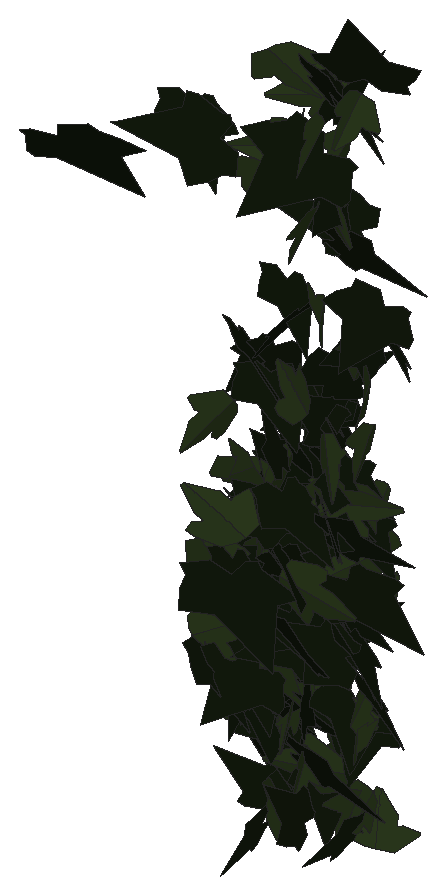
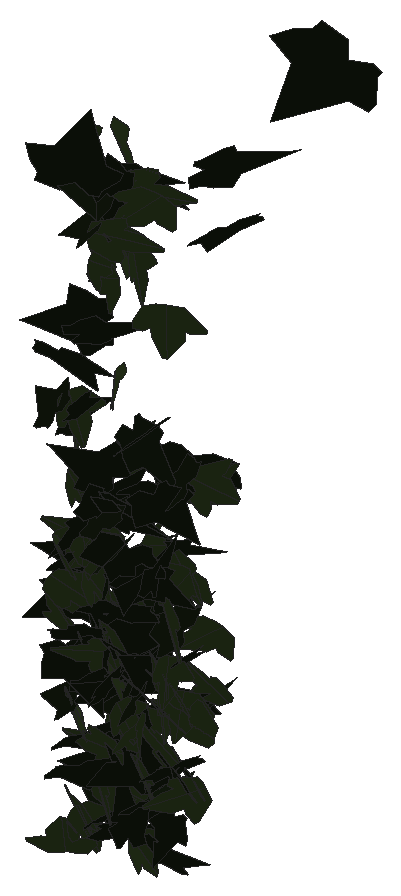
# SketchUp Ruby script. Lengths in inches.
U = 1.inch
M = Sketchup.active_model
def pt(a) = Geom::Point3d.new(a.map { |v| v * U })
def face(e, loops, mat)
  f = e.add_face(loops[0].map { |a| pt(a) })
  loops[1..].each { |l| e.add_face(l.map { |a| pt(a) }).erase! }
  f.material = f.back_material = mat if mat
  f
end
# faces: each face lists its corners as indices into pts; further lists are holes
def faces(e, pts, list, mat = nil) = list.each { |f| face(e, (f[0].is_a?(Array) ? f : [f]).map { |l| l.map { |i| pts[i] } }, mat) }
# xy, xz, yz: faces in a plane at the given z, y or x. An outline is a flat list of corners, or four numbers for a rectangle; further outlines are holes
def ring(l) = l.size == 4 ? [[l[0], l[1]], [l[2], l[1]], [l[2], l[3]], [l[0], l[3]]] : l.each_slice(2).to_a
def flat(e, list, mat, &to3) = list.each { |f| face(e, (f[0].is_a?(Array) ? f : [f]).map { |l| ring(l).map { |u, v| to3.(u, v) } }, mat) }
def xy(e, z, list, mat = nil) = flat(e, list, mat) { |x, y| [x, y, z] }
def xz(e, y, list, mat = nil) = flat(e, list, mat) { |x, z| [x, y, z] }
def yz(e, x, list, mat = nil) = flat(e, list, mat) { |y, z| [x, y, z] }
def lines(e, pts, list) = list.each { |a, b| e.add_line(pt(pts[a]), pt(pts[b])) }
# prism: a flat outline (further loops are holes) pulled along v
def prism(e, loops, v, mat = nil)
  f = face(e, loops, mat); d = Geom::Vector3d.new(v.map { |x| x * U })
  f.pushpull(f.normal.samedirection?(d) ? d.length : -d.length)
end
def box(e, o, s, mat = nil) = prism(e, [[o, [o[0] + s[0], o[1], o[2]], [o[0] + s[0], o[1] + s[1], o[2]], [o[0], o[1] + s[1], o[2]]]], [0, 0, s[2]], mat)
def at(x, y, z, deg = 0) = Geom::Transformation.translation(pt([x, y, z])) * Geom::Transformation.rotation(ORIGIN, Z_AXIS, deg.degrees)
def axes(o, x, y, z) = Geom::Transformation.new([*x, 0, *y, 0, *z, 0, *pt(o).to_a, 1])
def part(name) = M.definitions.add(name)
# library, detail: a bought-in or finely detailed component or shape, given as its bounding box
def library(name, o, s) = part(name).tap { |d| box(d.entities, o, s) }
def detail(e, o, s) = box(e.add_group.entities, o, s)
def put(e, d, t, mat = nil) = e.add_instance(d, t).tap { |i| i.material = mat if mat }
def group(e, t, mat = nil) = e.add_group.tap { |g| g.transformation = t; g.material = mat if mat }.entities
root = M.entities
M.materials.add("1026 AP 7946 SUNNY SIDE UP").color = [254, 231, 186]
M.materials.add("efeu1").color = [18, 25, 13]
M.materials.add("efeu2").color = [43, 57, 29]
c1 = part("ivyleaf_9")
p = [[1.54,2.16,1.25],[1.36,2.04,1.19],[-0.21,0.99,0.68],[-0.71,1.11,0.82],[-0.85,0.86,0.67],[-0.8,0.17,0.21],
  [-0.9,-0.01,0.1],[-0.67,-0.16,-0.02],[-0.08,-0.08,-0.05],[-0.03,-0.6,-0.4],[0.65,-0.88,-0.66],[0.83,-0.6,-0.49],
  [1.29,-0.42,-0.43],[1.8125,-0.07,-0.26],[1.21,0.44,0.15]]
faces(c1.entities,p,[[0,1,2,3,4,5,6,7,8,9,10,11,12,13,14]],"efeu1")
c2 = part("ivyleaf_10")
p = [[0,0.5,-0.03],[-0.0625,2.02,-0.43],[-0.19,2.01,-0.46],[-0.54,1.05,-0.29],[-0.52,0.625,-0.18],[-0.83,0.76,-0.28],
  [-1.16,0.64,-0.33],[-1.15,0.33,-0.24],[-0.77,-0.39,0.02],[-0.3,-0.51,0.16],[0.04,-0.48,0.23],[-0.02,2.01,-0.4375],
  [-0.06,2.01,-0.43],[0.04,-0.49,0.23],[0.67,-0.49,0.14],[1.38,0.36,-0.2],[1.375,0.51,-0.24],[0.81,0.65,-0.19],
  [0.62,0.59,-0.15],[0.6,1.09,-0.28],[0.5,1.23,-0.31]]
faces(c2.entities,p,[[0,1,2,3,4,5,6,7,8,9,10],[11,12,0,13,14,15,16,17,18,19,20]],"efeu2")
put(root,c1,axes([119.4375,207.16,279.6],[0.64011,0.19649,0.04423],[0.08407,-0.01489,-0.46425],[-0.30449,0.40896,-0.03521]),"1026 AP 7946 SUNNY SIDE UP")
put(root,c1,axes([121.18,208.625,272.82],[-0.2498,-0.24915,-0.28445],[0.28289,0.20954,-0.30176],[0.50992,-0.2383,0.02806]),"1026 AP 7946 SUNNY SIDE UP")
put(root,c1,axes([120,209.72,278.67],[-0.11484,-0.29306,-0.27056],[-0.04005,-0.26135,0.30816],[-0.61573,0.07166,0.03042]),"1026 AP 7946 SUNNY SIDE UP")
put(root,c2,axes([120.375,209.6,272.92],[0.1763,0.27302,0.20783],[-0.16656,-0.172,0.30177],[0.50561,-0.15186,0.02694]),"1026 AP 7946 SUNNY SIDE UP")
put(root,c1,axes([120.57,209.97,268.24],[-0.30854,0.13802,-0.17309],[0.19369,-0.11721,-0.24693],[-0.28291,-0.23078,0.01971]),"1026 AP 7946 SUNNY SIDE UP")
put(root,c1,axes([121.38,209.85,268.64],[-0.23324,0.03837,-0.26203],[-0.39193,0.05209,0.15802],[0.10126,0.28999,0.00807]),"1026 AP 7946 SUNNY SIDE UP")
put(root,c2,axes([121.3,210.23,278.98],[0.25906,-0.33094,0.02563],[-0.00335,-0.03092,-0.38068],[0.52205,0.16402,-0.01516]),"1026 AP 7946 SUNNY SIDE UP")
put(root,c1,axes([121.22,210.41,278.53],[-0.6117,-0.16424,0.04847],[-0.04205,-0.05935,-0.433],[0.26574,-0.38745,0.04306]),"1026 AP 7946 SUNNY SIDE UP")
put(root,c1,axes([120.72,210.45,270.88],[0.44713,-0.21603,-0.03017],[0.07123,0.01351,0.36588],[-0.33506,-0.28542,0.03753]),"1026 AP 7946 SUNNY SIDE UP")
put(root,c2,axes([119.36,210.64,273.88],[-0.05934,-0.20383,0.30376],[0.01008,-0.29797,-0.21228],[0.56504,-0.01609,0.03569]),"1026 AP 7946 SUNNY SIDE UP")
put(root,c1,axes([118.96,210.57,278.4],[-0.01902,-0.35708,-0.05764],[0.02386,0.0534,-0.36751],[0.56734,-0.01421,0.01352]),"1026 AP 7946 SUNNY SIDE UP")
put(root,c2,axes([120.8,210.6,278.43],[0.12113,-0.00994,-0.36126],[-0.50129,-0.15168,-0.06861],[-0.22999,0.32536,-0.04071]),"1026 AP 7946 SUNNY SIDE UP")
put(root,c1,axes([119.21,210.53,270.18],[0.23736,-0.30645,-0.08631],[-0.0673,0.07035,-0.35144],[0.49426,0.15674,-0.00641]),"1026 AP 7946 SUNNY SIDE UP")
put(root,c2,axes([120.92,210.58,277.41],[0.12282,-0.35113,0.0529],[0.00072,-0.05452,-0.37071],[0.55845,0.07729,-0.01116]),"1026 AP 7946 SUNNY SIDE UP")
put(root,c1,axes([120.16,210.72,272.51],[-0.31823,-0.07491,0.20229],[-0.24417,-0.13125,-0.21676],[0.22361,-0.24992,0.05121]),"1026 AP 7946 SUNNY SIDE UP")
put(root,c1,axes([119.85,210.78,270.01],[-0.35023,-0.24723,0.12467],[-0.09219,-0.11132,-0.34216],[0.42389,-0.22848,0.02859]),"1026 AP 7946 SUNNY SIDE UP")
put(root,c1,axes([119.58,210.65,271.62],[0.14268,-0.32554,-0.02877],[-0.02831,0.02203,-0.34782],[0.51273,0.09181,-0.0112]),"1026 AP 7946 SUNNY SIDE UP")
put(root,c2,axes([120.18,210.71,268.08],[-0.06528,0.01007,0.34132],[0.46943,-0.14382,0.04221],[0.22626,0.30129,0.01091]),"1026 AP 7946 SUNNY SIDE UP")
put(root,c2,axes([119.07,210.66,270.38],[0.2878,-0.07638,-0.21473],[0.32018,-0.0484,0.20262],[-0.13739,-0.2728,0.0224]),"1026 AP 7946 SUNNY SIDE UP")
put(root,c1,axes([121.5,210.73,268.11],[-0.29188,0.21127,-0.08709],[0.06606,-0.07698,-0.28956],[-0.35238,-0.18943,0.01786]),"1026 AP 7946 SUNNY SIDE UP")
put(root,c1,axes([121.22,210.89,270.65],[-0.19629,-0.25938,-0.14117],[-0.10751,-0.11745,0.2957],[-0.44746,0.142,-0.00912]),"1026 AP 7946 SUNNY SIDE UP")
put(root,c2,axes([121.47,210.93,279.14],[0.1149,0.22617,-0.21797],[-0.11951,-0.19901,-0.24588],[-0.47353,0.10511,0.00916]),"1026 AP 7946 SUNNY SIDE UP")
put(root,c2,axes([120.43,210.94,271.45],[-0.08234,-0.00073,-0.36593],[0.50214,-0.15729,-0.04909],[-0.24453,-0.32275,0.02241]),"1026 AP 7946 SUNNY SIDE UP")
put(root,c2,axes([119.01,210.85,271.5625],[-0.34863,-0.0415,-0.18311],[0.28597,-0.03129,-0.22667],[0.01955,-0.28229,0.05033]),"1026 AP 7946 SUNNY SIDE UP")
put(root,c2,axes([120.5,211.07,268.74],[-0.00229,0.18835,-0.23483],[-0.03553,-0.22843,-0.19472],[-0.4649,0.01653,0.01604]),"1026 AP 7946 SUNNY SIDE UP")
put(root,c1,axes([120.18,211.18,271.46],[0.02218,-0.19522,0.24221],[0.04846,-0.23437,-0.20281],[0.47942,0.03272,0.00929]),"1026 AP 7946 SUNNY SIDE UP")
put(root,c1,axes([120.49,211.01,268.78],[0.41517,-0.14986,0.1736],[0.20888,-0.10793,-0.31236],[0.28779,0.29454,-0.02373]),"1026 AP 7946 SUNNY SIDE UP")
put(root,c1,axes([120.17,211,272.71],[0.10327,-0.28964,-0.14862],[0.0423,0.14994,-0.30007],[0.50588,0.04659,0.05543]),"1026 AP 7946 SUNNY SIDE UP")
put(root,c1,axes([120.79,211.26,277.42],[-0.05716,-0.2167,0.2424],[-0.07041,-0.23229,-0.22769],[0.49947,-0.05755,-0.00435]),"1026 AP 7946 SUNNY SIDE UP")
put(root,c1,axes([120.33,210.96,270.93],[-0.04795,-0.1826,-0.27679],[0.16866,0.24798,-0.18543],[0.48073,-0.10521,0.03745]),"1026 AP 7946 SUNNY SIDE UP")
put(root,c1,axes([120.6,210.89,269.82],[0.13315,-0.0998,-0.30264],[-0.38165,0.16745,-0.12995],[0.30254,0.25515,-0.03073]),"1026 AP 7946 SUNNY SIDE UP")
put(root,c1,axes([120.33,211.26,270.32],[-0.32033,-0.06908,0.19298],[-0.23628,-0.12399,-0.21573],[0.20759,-0.24772,0.05224]),"1026 AP 7946 SUNNY SIDE UP")
put(root,c2,axes([120.28,211.14,274.1],[-0.12262,0.3353,0.09688],[0.03475,-0.08945,0.35411],[0.54566,0.08105,-0.00078]),"1026 AP 7946 SUNNY SIDE UP")
put(root,c2,axes([119.85,211.36,272.93],[-0.00582,-0.10664,0.29579],[0.15438,-0.27303,-0.10454],[0.45713,0.09085,0.03907]),"1026 AP 7946 SUNNY SIDE UP")
put(root,c1,axes([120.02,211.09,273.11],[-0.06759,-0.19878,0.2134],[0.06101,0.20466,0.21067],[-0.44857,0.05779,-0.0035]),"1026 AP 7946 SUNNY SIDE UP")
put(root,c1,axes([121.05,211.34,270.72],[0.15408,-0.29961,0.11538],[0.04377,-0.11049,-0.3253],[0.50199,0.1016,-0.00705]),"1026 AP 7946 SUNNY SIDE UP")
put(root,c2,axes([118.94,211.18,270.03],[-0.11812,0.03059,0.32267],[0.49236,0.03765,0.07384],[-0.04668,0.31972,-0.03766]),"1026 AP 7946 SUNNY SIDE UP")
put(root,c2,axes([120.72,211.24,273.5],[-0.05027,0.30861,-0.12351],[0.0161,-0.12123,-0.32033],[-0.52135,-0.0335,0.00201]),"1026 AP 7946 SUNNY SIDE UP")
put(root,c1,axes([120.85,211.18,272.24],[0.27653,-0.0414,0.23212],[0.3306,-0.08437,-0.18534],[0.14396,0.27329,-0.02026]),"1026 AP 7946 SUNNY SIDE UP")
put(root,c2,axes([121.45,211.01,269.3],[0.18976,-0.01338,0.28389],[-0.28825,0.22099,0.09503],[-0.32436,-0.20422,0.08163]),"1026 AP 7946 SUNNY SIDE UP")
put(root,c2,axes([120.59,211.35,277.32],[-0.23857,0.14319,-0.30052],[0.26092,-0.2437,-0.21298],[-0.44066,-0.22181,0.03659]),"1026 AP 7946 SUNNY SIDE UP")
put(root,c1,axes([119.21,211.33,269.41],[-0.29558,0.03267,-0.2119],[0.3095,-0.06345,-0.19589],[-0.10792,-0.27147,0.01858]),"1026 AP 7946 SUNNY SIDE UP")
put(root,c2,axes([119.3,211.2,270.4],[-0.21866,-0.25678,-0.08166],[0.07961,0.06094,-0.30008],[0.41431,-0.14723,0.01457]),"1026 AP 7946 SUNNY SIDE UP")
put(root,c2,axes([120.15,211.23,269.89],[-0.36567,-0.16282,-0.05275],[0.09054,0.00498,-0.29095],[0.25219,-0.23787,0.02797]),"1026 AP 7946 SUNNY SIDE UP")
put(root,c2,axes([120.68,211.3,268.54],[-0.07939,0.00442,0.3361],[-0.47884,-0.11911,-0.04759],[0.1841,-0.30788,0.02116]),"1026 AP 7946 SUNNY SIDE UP")
put(root,c2,axes([121.41,211.17,274.67],[0.17665,-0.29258,-0.17413],[-0.02271,0.17208,-0.31887],[0.52951,0.10498,0.04442]),"1026 AP 7946 SUNNY SIDE UP")
put(root,c1,axes([121.11,211.22,271.57],[-0.04231,-0.13448,-0.32939],[0.31919,0.25302,-0.12606],[0.44089,-0.19608,0.05965]),"1026 AP 7946 SUNNY SIDE UP")
put(root,c2,axes([119.41,211.2,272.74],[-0.27485,0.08401,0.22022],[-0.33915,0.0306,-0.19433],[-0.12212,-0.27406,0.04404]),"1026 AP 7946 SUNNY SIDE UP")
put(root,c1,axes([120.52,211.48,272.27],[0.17272,-0.11366,-0.29179],[0.40349,-0.12732,0.15476],[-0.25803,-0.27517,0.04669]),"1026 AP 7946 SUNNY SIDE UP")
put(root,c1,axes([119.43,211.49,268.87],[-0.04965,-0.24922,0.15905],[0.08834,-0.15892,-0.2511],[0.45363,0.00367,0.06631]),"1026 AP 7946 SUNNY SIDE UP")
put(root,c1,axes([119.91,211.42,270],[-0.01284,0.07379,0.29121],[0.08932,-0.27656,0.07456],[0.44995,0.057,-0.00649]),"1026 AP 7946 SUNNY SIDE UP")
put(root,c1,axes([119.21,211.54,271.17],[-0.14463,-0.16825,0.21201],[-0.1172,-0.19375,-0.19773],[0.40242,-0.1169,0.01861]),"1026 AP 7946 SUNNY SIDE UP")
put(root,c1,axes([120.52,211.12,271.02],[0.29042,0.10657,0.20357],[0.26311,0.10408,-0.21902],[-0.2341,0.24918,0.00639]),"1026 AP 7946 SUNNY SIDE UP")
put(root,c1,axes([120.45,211.5,268.22],[-0.0512,-0.29728,0.05161],[-0.0025,-0.05192,-0.30836],[0.47448,-0.03235,0.00395]),"1026 AP 7946 SUNNY SIDE UP")
put(root,c2,axes([120.72,211.29,270.8125],[0.30897,-0.12041,-0.18282],[-0.23315,0.09632,-0.23682],[0.24239,0.24613,0.00525]),"1026 AP 7946 SUNNY SIDE UP")
put(root,c2,axes([119.86,211.48,269.14],[0.21241,-0.18019,0.19882],[0.1691,-0.16169,-0.23279],[0.38045,0.17247,-0.00753]),"1026 AP 7946 SUNNY SIDE UP")
put(root,c1,axes([121.17,211.46,269.97],[0.22785,-0.24521,0.1034],[0.05415,-0.09759,-0.29335],[0.41392,0.14775,-0.01854]),"1026 AP 7946 SUNNY SIDE UP")
put(root,c1,axes([121.4375,211.47,275.78],[-0.48833,-0.10453,-0.08411],[0.13606,-0.0041,-0.33613],[0.15731,-0.32094,0.02962]),"1026 AP 7946 SUNNY SIDE UP")
put(root,c1,axes([119.11,211.49,271.83],[0.26589,-0.26432,0.15599],[0.11306,-0.13542,-0.32385],[0.46666,0.18341,-0.01042]),"1026 AP 7946 SUNNY SIDE UP")
put(root,c1,axes([120.07,211.43,271.55],[-0.01114,0.17394,-0.26746],[-0.01895,-0.26063,-0.18039],[-0.4923,0.0061,0.013]),"1026 AP 7946 SUNNY SIDE UP")
put(root,c2,axes([120.86,211.49,272.7],[-0.2277,-0.12269,0.22405],[-0.16869,-0.19732,-0.18881],[0.35561,-0.17216,0.05389]),"1026 AP 7946 SUNNY SIDE UP")
put(root,c2,axes([121.15,211.52,271.86],[-0.19099,-0.10629,0.25079],[-0.1731,-0.22418,-0.15834],[0.38108,-0.1551,0.05377]),"1026 AP 7946 SUNNY SIDE UP")
put(root,c2,axes([119.16,211.34,272.65],[-0.40349,-0.06601,-0.11384],[0.18374,-0.01809,-0.26944],[0.08365,-0.27866,0.04272]),"1026 AP 7946 SUNNY SIDE UP")
put(root,c1,axes([120.1,211.62,270.94],[-0.17913,-0.22293,0.19442],[-0.06849,-0.18869,-0.25611],[0.45545,-0.11606,0.03795]),"1026 AP 7946 SUNNY SIDE UP")
put(root,c2,axes([121.16,211.51,273.74],[0.03832,-0.25995,0.1597],[0.11783,-0.14698,-0.2644],[0.46232,0.05901,0.05415]),"1026 AP 7946 SUNNY SIDE UP")
put(root,c1,axes([119.6,211.44,274.125],[-0.09381,-0.28636,-0.13463],[0.08169,0.12056,-0.29962],[0.48709,-0.07537,0.02432]),"1026 AP 7946 SUNNY SIDE UP")
put(root,c2,axes([119.36,211.49,269.59],[0.15757,-0.11187,-0.28867],[0.3501,-0.17084,0.15165],[-0.31877,-0.24293,0.02386]),"1026 AP 7946 SUNNY SIDE UP")
put(root,c1,axes([120.32,211.49,278.89],[0.32705,-0.17635,0.19512],[0.19277,-0.1483,-0.28034],[0.35968,0.23984,-0.02717]),"1026 AP 7946 SUNNY SIDE UP")
put(root,c2,axes([120.72,211.31,272.61],[-0.17793,-0.04388,0.34492],[0.4662,0.15663,0.12521],[-0.25492,0.31707,-0.01177]),"1026 AP 7946 SUNNY SIDE UP")
put(root,c2,axes([120.59,211.17,275.48],[0.10843,-0.02907,-0.32005],[-0.07505,0.31327,-0.0393],[0.48459,0.05502,0.06552]),"1026 AP 7946 SUNNY SIDE UP")
put(root,c1,axes([120.07,211.35,272.45],[0.11809,-0.03329,-0.28648],[0.31214,0.20916,0.03068],[0.31022,-0.19778,0.07818]),"1026 AP 7946 SUNNY SIDE UP")
put(root,c2,axes([121.1,211.41,269.46],[0.32548,-0.2364,-0.0018],[0.02453,0.01312,0.3231],[-0.37091,-0.20658,0.01979]),"1026 AP 7946 SUNNY SIDE UP")
put(root,c1,axes([119.65,211.41,269.25],[0.36928,-0.05308,0.15599],[0.22159,-0.06122,-0.24714],[0.12157,0.27281,-0.02337]),"1026 AP 7946 SUNNY SIDE UP")
put(root,c2,axes([121.13,211.49,268.15],[0.36307,-0.23258,-0.01836],[-0.03593,0.00055,-0.33723],[0.36486,0.23149,-0.01493]),"1026 AP 7946 SUNNY SIDE UP")
put(root,c2,axes([119.96,211.46,269.22],[0.2691,-0.2142,-0.06571],[-0.07268,0.04311,-0.28204],[0.34327,0.17704,-0.00821]),"1026 AP 7946 SUNNY SIDE UP")
put(root,c2,axes([119.54,211.36,270.49],[0.04834,-0.2822,-0.17451],[-0.02735,0.16689,-0.29147],[0.51552,0.03532,0.0009]),"1026 AP 7946 SUNNY SIDE UP")
put(root,c1,axes([119.66,211.41,267.76],[-0.0692,0.09627,0.25635],[-0.35165,0.12326,-0.08935],[-0.22732,-0.21998,0.06018]),"1026 AP 7946 SUNNY SIDE UP")
put(root,c1,axes([120.84,211.65,269.51],[-0.1307,-0.32295,0.0199],[0.00433,-0.02254,-0.34357],[0.50888,-0.08275,0.00803]),"1026 AP 7946 SUNNY SIDE UP")
put(root,c1,axes([118.94,211.61,274.45],[0.25807,-0.26511,0.0809],[0.03312,-0.08082,-0.32075],[0.43419,0.16374,-0.02362]),"1026 AP 7946 SUNNY SIDE UP")
put(root,c1,axes([119.1875,211.6,269.49],[-0.04094,-0.29664,-0.0478],[0.01499,0.04404,-0.30646],[0.47147,-0.02716,0.00559]),"1026 AP 7946 SUNNY SIDE UP")
put(root,c1,axes([120.77,211.69,270.27],[-0.17243,-0.0405,0.29921],[-0.39356,-0.14912,-0.11955],[0.24095,-0.27254,0.01885]),"1026 AP 7946 SUNNY SIDE UP")
put(root,c1,axes([120.7,211.5,276.53],[0.42187,-0.06994,0.18928],[0.25874,-0.0914,-0.28331],[0.1702,0.3123,-0.03846]),"1026 AP 7946 SUNNY SIDE UP")
put(root,c1,axes([120.83,211.39,273.07],[0.08353,-0.13252,-0.26085],[-0.04929,0.25253,-0.14188],[0.44561,0.05277,0.0332]),"1026 AP 7946 SUNNY SIDE UP")
put(root,c2,axes([120.91,211.61,268.05],[-0.10393,-0.27534,0.1018],[0.00138,-0.10308,-0.29131],[0.46081,-0.06179,0.02383]),"1026 AP 7946 SUNNY SIDE UP")
put(root,c1,axes([121,211.76,274.99],[0.01931,-0.15264,-0.25933],[0.16254,-0.23277,0.14976],[-0.43219,-0.09436,0.04474]),"1026 AP 7946 SUNNY SIDE UP")
put(root,c1,axes([121.09,211.51,272.41],[0.05059,-0.23177,-0.17814],[-0.05518,0.16824,-0.23988],[0.45009,0.04668,-0.00938]),"1026 AP 7946 SUNNY SIDE UP")
put(root,c1,axes([119.1875,211.64,269.49],[-0.31572,0.01068,-0.1992],[0.29626,-0.05396,-0.20488],[-0.07078,-0.27352,0.03098]),"1026 AP 7946 SUNNY SIDE UP")
put(root,c2,axes([120.19,211.72,270.89],[0.15246,-0.24494,0.21353],[0.14067,-0.18882,-0.27227],[0.48601,0.13149,0.01182]),"1026 AP 7946 SUNNY SIDE UP")
put(root,c2,axes([119.79,211.67,267.98],[0.04435,-0.2655,0.13493],[0.02215,-0.13174,-0.27583],[0.46604,0.03153,0.00027]),"1026 AP 7946 SUNNY SIDE UP")
put(root,c2,axes([119.36,211.55,277.17],[-0.42915,-0.16208,0.01306],[0.00313,-0.02989,-0.32603],[0.25573,-0.27163,0.02591]),"1026 AP 7946 SUNNY SIDE UP")
put(root,c2,axes([120.87,211.53,272.78],[-0.43203,0.01978,-0.09096],[0.13556,-0.02961,-0.28303],[-0.04375,-0.28711,0.02122]),"1026 AP 7946 SUNNY SIDE UP")
put(root,c1,axes([120.02,211.51,268.15],[0.11017,-0.20398,-0.20724],[0.1226,0.21177,-0.19312],[0.43215,-0.00807,0.10762]),"1026 AP 7946 SUNNY SIDE UP")
put(root,c1,axes([119.28,211.48,268.53],[0.37338,-0.04979,-0.15099],[-0.23272,0.00377,-0.24881],[0.06981,0.27887,-0.02191]),"1026 AP 7946 SUNNY SIDE UP")
put(root,c1,axes([119.43,211.66,268.83],[-0.06684,-0.30938,-0.08809],[0.04966,0.08003,-0.32061],[0.50153,-0.04916,0.02]),"1026 AP 7946 SUNNY SIDE UP")
put(root,c2,axes([119.66,211.51,279],[-0.33517,-0.12472,-0.1997],[0.31041,0.0357,-0.248],[0.18529,-0.28542,0.05423]),"1026 AP 7946 SUNNY SIDE UP")
put(root,c2,axes([121.2,211.57,271.17],[0.35681,-0.1422,-0.10834],[0.16261,-0.03049,0.27429],[-0.22467,-0.2479,0.02646]),"1026 AP 7946 SUNNY SIDE UP")
put(root,c2,axes([120.49,211.79,277.79],[-0.00184,-0.16551,0.2853],[0.15051,-0.2656,-0.16412],[0.48578,0.08166,0.05193]),"1026 AP 7946 SUNNY SIDE UP")
put(root,c2,axes([119.9,211.5625,277.98],[0.04923,-0.32271,-0.06062],[0.01222,0.05799,-0.33341],[0.51515,0.02946,0.0137]),"1026 AP 7946 SUNNY SIDE UP")
put(root,c2,axes([120.64,211.73,272.3],[0.02821,-0.25241,0.16283],[0.05274,-0.15706,-0.26088],[0.46651,0.03302,0.01965]),"1026 AP 7946 SUNNY SIDE UP")
put(root,c2,axes([119.36,211.5,272.09],[0.24327,-0.24635,-0.20284],[-0.12362,0.18066,-0.29757],[0.47882,0.17181,0.02623]),"1026 AP 7946 SUNNY SIDE UP")
put(root,c2,axes([121.07,211.63,275.13],[-0.10701,-0.32584,0.02398],[0.00254,-0.02601,-0.343],[0.51387,-0.06773,0.00669]),"1026 AP 7946 SUNNY SIDE UP")
put(root,c1,axes([120.43,211.61,270.96],[0.03988,-0.05416,-0.28716],[0.39629,0.13258,-0.00214],[0.20467,-0.24616,0.0601]),"1026 AP 7946 SUNNY SIDE UP")
put(root,c1,axes([121.01,211.77,271.28],[-0.35243,-0.14893,0.06184],[-0.06191,-0.05045,-0.27677],[0.24529,-0.22671,0.019]),"1026 AP 7946 SUNNY SIDE UP")
put(root,c2,axes([120.36,211.65,269.41],[-0.0248,-0.02623,-0.29386],[0.42955,-0.08683,-0.00785],[-0.13473,-0.27201,0.02907]),"1026 AP 7946 SUNNY SIDE UP")
put(root,c1,axes([120.37,211.65,271.15],[-0.40195,0.09165,0.08886],[-0.14106,0.00262,-0.27841],[-0.13801,-0.26961,0.02574]),"1026 AP 7946 SUNNY SIDE UP")
put(root,c1,axes([119.71,211.77,272.64],[0.0242,0.01238,-0.29336],[-0.10683,-0.27687,-0.0178],[-0.43538,0.06862,-0.01194]),"1026 AP 7946 SUNNY SIDE UP")
put(root,c1,axes([119.46,211.74,272.56],[-0.00526,0.13011,0.26477],[-0.2649,-0.20853,0.10558],[0.36614,-0.149,0.08019]),"1026 AP 7946 SUNNY SIDE UP")
put(root,c1,axes([120.16,211.69,271.93],[-0.19304,-0.23875,-0.15667],[0.13201,0.12605,-0.27542],[0.42389,-0.14799,0.01442]),"1026 AP 7946 SUNNY SIDE UP")
put(root,c2,axes([118.9,211.45,269.09],[-0.1017,-0.09421,-0.31379],[0.34283,0.21295,-0.11451],[0.36468,-0.22646,0.02014]),"1026 AP 7946 SUNNY SIDE UP")
put(root,c1,axes([120.4375,211.8,273.5],[0.0477,0.0545,0.32889],[-0.40181,-0.19248,0.0578],[0.3121,-0.25612,0.02414]),"1026 AP 7946 SUNNY SIDE UP")
put(root,c1,axes([119.8125,211.6875,275.05],[-0.21954,0.25022,-0.2063],[0.12437,-0.18637,-0.29571],[-0.48979,-0.15948,0.01739]),"1026 AP 7946 SUNNY SIDE UP")
put(root,c1,axes([119.95,211.45,269.21],[0.25046,0.14517,0.17122],[0.18662,0.11525,-0.2213],[-0.29138,0.19859,0.00544]),"1026 AP 7946 SUNNY SIDE UP")
put(root,c1,axes([120.95,211.73,279.0625],[0.46895,0.00204,0.20875],[-0.31728,0.03607,0.3058],[-0.02924,-0.35875,0.02981]),"1026 AP 7946 SUNNY SIDE UP")
put(root,c2,axes([120.6,211.55,268.69],[0.15373,-0.18505,-0.19659],[-0.12168,0.17354,-0.21438],[0.39863,0.12434,0.01038]),"1026 AP 7946 SUNNY SIDE UP")
put(root,c1,axes([119.77,211.72,270.6875],[-0.41692,0.08296,-0.05004],[0.05864,-0.04408,-0.28474],[-0.13973,-0.26602,0.02982]),"1026 AP 7946 SUNNY SIDE UP")
put(root,c2,axes([119.2,211.83,271.07],[-0.10179,0.0364,-0.29458],[0.19304,-0.26191,-0.06446],[-0.41044,-0.1322,0.04274]),"1026 AP 7946 SUNNY SIDE UP")
put(root,c1,axes([119.61,211.46,270.85],[-0.08503,-0.03267,0.32226],[0.34197,0.22567,0.06429],[-0.35767,0.22353,-0.01514]),"1026 AP 7946 SUNNY SIDE UP")
put(root,c2,axes([120.4,211.68,271.45],[0.35188,-0.18157,-0.04222],[-0.03746,0.034,-0.29646],[0.28993,0.22477,0.01294]),"1026 AP 7946 SUNNY SIDE UP")
put(root,c1,axes([120.18,211.89,272.83],[-0.03582,-0.21804,0.1882],[-0.02739,-0.1831,-0.22691],[0.44769,-0.02865,0.00117]),"1026 AP 7946 SUNNY SIDE UP")
put(root,c2,axes([119.05,211.68,270.71],[0.4193,-0.19363,-0.09173],[0.1419,-0.02469,0.33776],[-0.3028,-0.2797,0.03126]),"1026 AP 7946 SUNNY SIDE UP")
put(root,c1,axes([120.68,211.44,278.52],[-0.24229,0.31542,-0.06554],[-0.03355,0.06235,0.36191],[0.5054,0.15535,-0.00739]),"1026 AP 7946 SUNNY SIDE UP")
put(root,c1,axes([120.29,211.79,273.8125],[-0.44967,0.01301,0.03816],[-0.06007,-0.03178,-0.29311],[-0.01375,-0.2866,0.03253]),"1026 AP 7946 SUNNY SIDE UP")
put(root,c2,axes([119.77,211.79,270.03],[0.04588,0.28064,-0.14075],[-0.02914,-0.13702,-0.29145],[-0.49103,0.03435,0.00415]),"1026 AP 7946 SUNNY SIDE UP")
put(root,c1,axes([120.29,211.97,270.54],[-0.13451,-0.07701,0.30835],[-0.22526,-0.26581,-0.11402],[0.43135,-0.16283,0.0366]),"1026 AP 7946 SUNNY SIDE UP")
put(root,c2,axes([120.42,211.6,271.03],[0.0867,-0.07582,-0.31068],[0.42588,0.16137,0.01018],[0.23887,-0.26017,0.09461]),"1026 AP 7946 SUNNY SIDE UP")
put(root,c1,axes([119.75,211.84,270.53],[0.26045,-0.22545,0.06112],[0.02988,-0.06105,-0.2878],[0.36587,0.16548,-0.02001]),"1026 AP 7946 SUNNY SIDE UP")
put(root,c1,axes([120.67,211.9,276.55],[-0.19782,0.03649,0.29422],[-0.42784,-0.11633,-0.10893],[0.14704,-0.28938,0.07889]),"1026 AP 7946 SUNNY SIDE UP")
put(root,c1,axes([120.99,211.73,270.9],[0.03525,0.2698,-0.17417],[-0.0395,-0.16899,-0.27973],[-0.50037,0.03235,0.00981]),"1026 AP 7946 SUNNY SIDE UP")
put(root,c1,axes([119.77,211.95,268.29],[-0.15857,0.00492,0.34251],[0.11821,-0.33806,0.02667],[0.50925,0.08,0.10046]),"1026 AP 7946 SUNNY SIDE UP")
put(root,c1,axes([120.69,211.9375,269.125],[-0.2332,-0.30201,-0.02568],[0.02926,0.01672,-0.34639],[0.47538,-0.14918,0.00872]),"1026 AP 7946 SUNNY SIDE UP")
put(root,c2,axes([121.1,211.86,272.09],[-0.20443,-0.04159,0.26032],[-0.33283,-0.14254,-0.13707],[0.22733,-0.24609,0.03343]),"1026 AP 7946 SUNNY SIDE UP")
put(root,c1,axes([119.96,211.69,272.97],[0.37431,0.14855,-0.15917],[-0.18874,-0.10042,-0.289],[-0.28037,0.26593,-0.01796]),"1026 AP 7946 SUNNY SIDE UP")
put(root,c1,axes([121.16,211.97,275.09],[0.08803,-0.20344,0.20828],[0.08413,-0.19617,-0.21852],[0.44439,0.07744,0.00011]),"1026 AP 7946 SUNNY SIDE UP")
put(root,c2,axes([121.1,211.89,272.65],[0.28464,-0.2123,0.07423],[0.05041,-0.0687,-0.28713],[0.34953,0.1828,-0.01904]),"1026 AP 7946 SUNNY SIDE UP")
put(root,c1,axes([119.26,211.89,274.25],[0.0243,0.14748,-0.2655],[-0.01527,-0.25851,-0.15402],[-0.46779,0.0161,-0.00877]),"1026 AP 7946 SUNNY SIDE UP")
put(root,c2,axes([120.21,211.96,278.42],[-0.08779,0.01745,0.32808],[-0.33279,-0.24376,-0.02589],[0.37497,-0.21226,0.05383]),"1026 AP 7946 SUNNY SIDE UP")
put(root,c1,axes([120.37,211.9,278.65],[0.28178,-0.28299,0.01837],[-0.00678,-0.02571,-0.34476],[0.44597,0.17841,-0.01685]),"1026 AP 7946 SUNNY SIDE UP")
put(root,c2,axes([119.12,211.76,271.31],[-0.09215,-0.2808,-0.10512],[0.0634,0.09396,-0.29431],[0.46463,-0.06851,0.01931]),"1026 AP 7946 SUNNY SIDE UP")
put(root,c1,axes([120.375,211.79,273.56],[-0.25011,0.09999,0.22807],[-0.3282,0.0778,-0.19073],[-0.1938,-0.26078,0.02866]),"1026 AP 7946 SUNNY SIDE UP")
put(root,c1,axes([119.45,211.96,275.28],[0.05688,-0.3231,0.01276],[-0.00613,-0.01475,-0.33497],[0.5085,0.03596,-0.00547]),"1026 AP 7946 SUNNY SIDE UP")
put(root,c2,axes([121.14,211.73,267.51],[0.40041,0.16102,-0.04284],[0.03033,0.04861,0.30907],[0.26009,-0.25355,0.02991]),"1026 AP 7946 SUNNY SIDE UP")
put(root,c1,axes([120.17,212.04,273.49],[-0.03734,-0.18865,0.2406],[0.10178,-0.23304,-0.18766],[0.46231,0.03607,0.06074]),"1026 AP 7946 SUNNY SIDE UP")
put(root,c2,axes([119.875,211.9375,270.35],[-0.06952,-0.26389,0.10058],[0.04505,-0.10403,-0.27273],[0.44095,-0.03098,0.04372]),"1026 AP 7946 SUNNY SIDE UP")
put(root,c1,axes([120.3125,211.7,274.16],[-0.03016,-0.00386,0.31114],[0.45463,0.0874,0.02057],[-0.13754,0.28976,-0.00022]),"1026 AP 7946 SUNNY SIDE UP")
